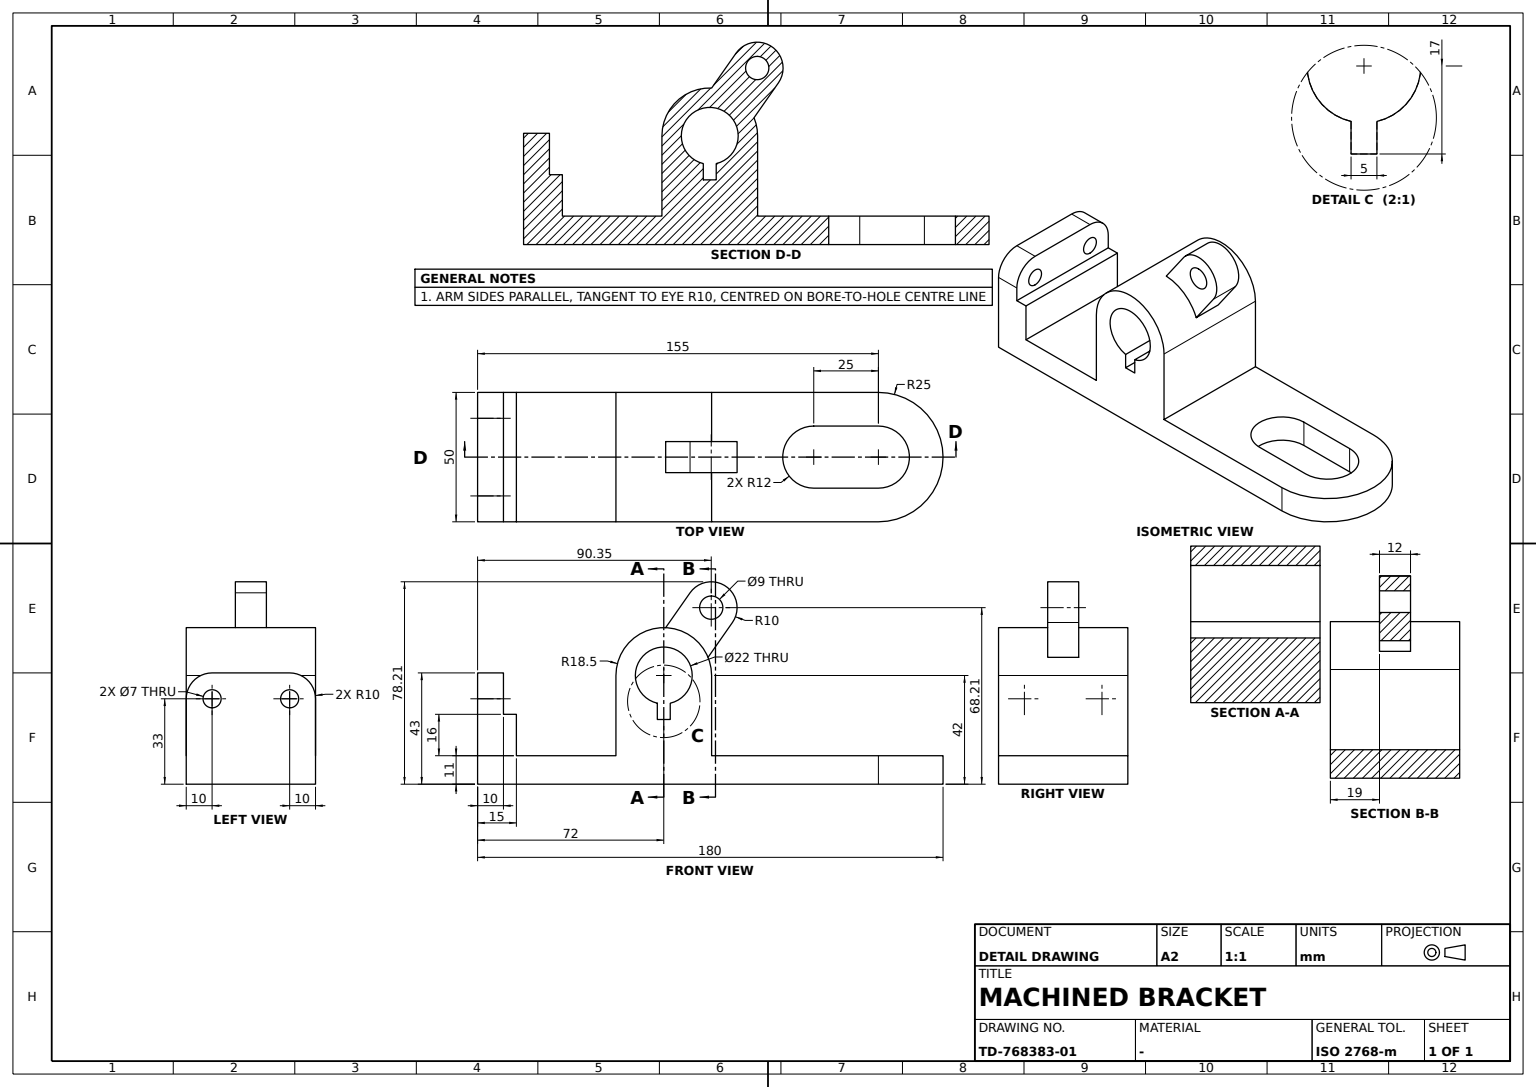
ISO-10303-21;
HEADER;
FILE_DESCRIPTION((''),'2;1');
FILE_NAME('','',(''),(''),'','','');
FILE_SCHEMA(('AUTOMOTIVE_DESIGN'));
ENDSEC;
DATA;
#1=APPLICATION_CONTEXT('');
#2=PRODUCT_CONTEXT('',#1,'mechanical');
#3=PRODUCT('','','',(#2));
#4=PRODUCT_DEFINITION_FORMATION('','',#3);
#5=PRODUCT_DEFINITION_CONTEXT('',#1,'design');
#6=PRODUCT_DEFINITION('','',#4,#5);
#7=PRODUCT_DEFINITION_SHAPE('','',#6);
#8=(LENGTH_UNIT()NAMED_UNIT(*)SI_UNIT(.MILLI.,.METRE.));
#9=(NAMED_UNIT(*)PLANE_ANGLE_UNIT()SI_UNIT($,.RADIAN.));
#10=(NAMED_UNIT(*)SI_UNIT($,.STERADIAN.)SOLID_ANGLE_UNIT());
#11=UNCERTAINTY_MEASURE_WITH_UNIT(LENGTH_MEASURE(0.005),#8,'distance_accuracy_value','');
#12=(GEOMETRIC_REPRESENTATION_CONTEXT(3)GLOBAL_UNCERTAINTY_ASSIGNED_CONTEXT((#11))GLOBAL_UNIT_ASSIGNED_CONTEXT((#8,#9,#10))REPRESENTATION_CONTEXT('',''));
#13=CARTESIAN_POINT('',(-77.5,15.,37.5));
#14=VERTEX_POINT('',#13);
#15=CARTESIAN_POINT('',(-77.5,25.,27.5));
#16=VERTEX_POINT('',#15);
#17=CARTESIAN_POINT('',(-77.5,15.,27.5));
#18=DIRECTION('',(1.,0.,0.));
#19=DIRECTION('',(0.,0.,-1.));
#20=AXIS2_PLACEMENT_3D('',#17,#18,#19);
#21=CIRCLE('',#20,10.);
#22=EDGE_CURVE('',#14,#16,#21,.F.);
#23=ORIENTED_EDGE('',*,*,#22,.F.);
#24=CARTESIAN_POINT('',(-67.5,15.,37.5));
#25=VERTEX_POINT('',#24);
#26=CARTESIAN_POINT('',(-70.,15.,37.5));
#27=DIRECTION('',(-1.,0.,0.));
#28=VECTOR('',#27,1000.);
#29=LINE('',#26,#28);
#30=EDGE_CURVE('',#14,#25,#29,.F.);
#31=ORIENTED_EDGE('',*,*,#30,.T.);
#32=CARTESIAN_POINT('',(-67.5,25.,27.5));
#33=VERTEX_POINT('',#32);
#34=CARTESIAN_POINT('',(-67.5,15.,27.5));
#35=AXIS2_PLACEMENT_3D('',#34,#18,#19);
#36=CIRCLE('',#35,10.);
#37=EDGE_CURVE('',#33,#25,#36,.T.);
#38=ORIENTED_EDGE('',*,*,#37,.F.);
#39=CARTESIAN_POINT('',(-70.,25.,27.5));
#40=LINE('',#39,#28);
#41=EDGE_CURVE('',#16,#33,#40,.F.);
#42=ORIENTED_EDGE('',*,*,#41,.F.);
#43=EDGE_LOOP('',(#23,#31,#38,#42));
#44=FACE_BOUND('',#43,.T.);
#45=CARTESIAN_POINT('',(-70.,15.,27.5));
#46=DIRECTION('',(0.,-1.,0.));
#47=AXIS2_PLACEMENT_3D('',#45,#27,#46);
#48=CYLINDRICAL_SURFACE('',#47,10.);
#49=ADVANCED_FACE('',(#44),#48,.T.);
#50=CARTESIAN_POINT('',(-67.5,-15.,24.));
#51=VERTEX_POINT('',#50);
#52=CARTESIAN_POINT('',(-67.5,-15.,27.5));
#53=AXIS2_PLACEMENT_3D('',#52,#18,#19);
#54=CIRCLE('',#53,3.5);
#55=EDGE_CURVE('',#51,#51,#54,.T.);
#56=ORIENTED_EDGE('',*,*,#55,.F.);
#57=EDGE_LOOP('',(#56));
#58=FACE_BOUND('',#57,.T.);
#59=CARTESIAN_POINT('',(-67.5,15.,24.));
#60=VERTEX_POINT('',#59);
#61=CIRCLE('',#35,3.5);
#62=EDGE_CURVE('',#60,#60,#61,.T.);
#63=ORIENTED_EDGE('',*,*,#62,.F.);
#64=EDGE_LOOP('',(#63));
#65=FACE_BOUND('',#64,.T.);
#66=CARTESIAN_POINT('',(-67.5,-15.,37.5));
#67=VERTEX_POINT('',#66);
#68=CARTESIAN_POINT('',(-67.5,-25.,27.5));
#69=VERTEX_POINT('',#68);
#70=CIRCLE('',#53,10.);
#71=EDGE_CURVE('',#67,#69,#70,.T.);
#72=ORIENTED_EDGE('',*,*,#71,.T.);
#73=CARTESIAN_POINT('',(-67.5,-25.,21.5));
#74=VERTEX_POINT('',#73);
#75=CARTESIAN_POINT('',(-67.5,-25.,0.));
#76=DIRECTION('',(0.,0.,1.));
#77=VECTOR('',#76,1000.);
#78=LINE('',#75,#77);
#79=EDGE_CURVE('',#74,#69,#78,.T.);
#80=ORIENTED_EDGE('',*,*,#79,.F.);
#81=CARTESIAN_POINT('',(-67.5,25.,21.5));
#82=VERTEX_POINT('',#81);
#83=VECTOR('',#46,1000.);
#84=LINE('',#81,#83);
#85=EDGE_CURVE('',#82,#74,#84,.T.);
#86=ORIENTED_EDGE('',*,*,#85,.F.);
#87=CARTESIAN_POINT('',(-67.5,25.,0.));
#88=VECTOR('',#19,1000.);
#89=LINE('',#87,#88);
#90=EDGE_CURVE('',#33,#82,#89,.T.);
#91=ORIENTED_EDGE('',*,*,#90,.F.);
#92=ORIENTED_EDGE('',*,*,#37,.T.);
#93=DIRECTION('',(0.,1.,0.));
#94=VECTOR('',#93,1000.);
#95=LINE('',#24,#94);
#96=EDGE_CURVE('',#67,#25,#95,.T.);
#97=ORIENTED_EDGE('',*,*,#96,.F.);
#98=EDGE_LOOP('',(#72,#80,#86,#91,#92,#97));
#99=FACE_BOUND('',#98,.T.);
#100=CARTESIAN_POINT('',(-67.5,0.,0.));
#101=AXIS2_PLACEMENT_3D('',#100,#18,#93);
#102=PLANE('',#101);
#103=ADVANCED_FACE('',(#58,#65,#99),#102,.T.);
#104=CARTESIAN_POINT('',(-24.,25.,5.5));
#105=VERTEX_POINT('',#104);
#106=CARTESIAN_POINT('',(-24.,25.,36.5));
#107=VERTEX_POINT('',#106);
#108=CARTESIAN_POINT('',(-24.,25.,-5.5));
#109=LINE('',#108,#77);
#110=EDGE_CURVE('',#105,#107,#109,.T.);
#111=ORIENTED_EDGE('',*,*,#110,.F.);
#112=CARTESIAN_POINT('',(-24.,-25.,5.5));
#113=VERTEX_POINT('',#112);
#114=CARTESIAN_POINT('',(-24.,0.,5.5));
#115=LINE('',#114,#83);
#116=EDGE_CURVE('',#105,#113,#115,.T.);
#117=ORIENTED_EDGE('',*,*,#116,.T.);
#118=CARTESIAN_POINT('',(-24.,-25.,36.5));
#119=VERTEX_POINT('',#118);
#120=CARTESIAN_POINT('',(-24.,-25.,0.));
#121=LINE('',#120,#77);
#122=EDGE_CURVE('',#113,#119,#121,.T.);
#123=ORIENTED_EDGE('',*,*,#122,.T.);
#124=CARTESIAN_POINT('',(-24.,0.,36.5));
#125=LINE('',#124,#83);
#126=EDGE_CURVE('',#119,#107,#125,.F.);
#127=ORIENTED_EDGE('',*,*,#126,.T.);
#128=EDGE_LOOP('',(#111,#117,#123,#127));
#129=FACE_BOUND('',#128,.T.);
#130=CARTESIAN_POINT('',(-24.,-25.,-5.5));
#131=AXIS2_PLACEMENT_3D('',#130,#27,#76);
#132=PLANE('',#131);
#133=ADVANCED_FACE('',(#129),#132,.T.);
#134=ORIENTED_EDGE('',*,*,#62,.T.);
#135=EDGE_LOOP('',(#134));
#136=FACE_BOUND('',#135,.T.);
#137=CARTESIAN_POINT('',(-77.5,15.,24.));
#138=VERTEX_POINT('',#137);
#139=CIRCLE('',#20,3.5);
#140=EDGE_CURVE('',#138,#138,#139,.T.);
#141=ORIENTED_EDGE('',*,*,#140,.F.);
#142=EDGE_LOOP('',(#141));
#143=FACE_BOUND('',#142,.T.);
#144=CARTESIAN_POINT('',(-73.16,15.,27.5));
#145=AXIS2_PLACEMENT_3D('',#144,#18,#93);
#146=CYLINDRICAL_SURFACE('',#145,3.5);
#147=ADVANCED_FACE('',(#136,#143),#146,.F.);
#148=CARTESIAN_POINT('',(-77.5,-15.,24.));
#149=VERTEX_POINT('',#148);
#150=CARTESIAN_POINT('',(-77.5,-15.,27.5));
#151=AXIS2_PLACEMENT_3D('',#150,#18,#19);
#152=CIRCLE('',#151,3.5);
#153=EDGE_CURVE('',#149,#149,#152,.T.);
#154=ORIENTED_EDGE('',*,*,#153,.F.);
#155=EDGE_LOOP('',(#154));
#156=FACE_BOUND('',#155,.T.);
#157=ORIENTED_EDGE('',*,*,#55,.T.);
#158=EDGE_LOOP('',(#157));
#159=FACE_BOUND('',#158,.T.);
#160=CARTESIAN_POINT('',(-73.16,-15.,27.5));
#161=AXIS2_PLACEMENT_3D('',#160,#18,#93);
#162=CYLINDRICAL_SURFACE('',#161,3.5);
#163=ADVANCED_FACE('',(#156,#159),#162,.F.);
#164=CARTESIAN_POINT('',(-8.,-25.,25.787857));
#165=VERTEX_POINT('',#164);
#166=CARTESIAN_POINT('',(-8.,-25.,19.5));
#167=VERTEX_POINT('',#166);
#168=LINE('',#164,#88);
#169=EDGE_CURVE('',#165,#167,#168,.T.);
#170=ORIENTED_EDGE('',*,*,#169,.T.);
#171=CARTESIAN_POINT('',(-8.,25.,19.5));
#172=VERTEX_POINT('',#171);
#173=CARTESIAN_POINT('',(-8.,6.,19.5));
#174=LINE('',#173,#83);
#175=EDGE_CURVE('',#172,#167,#174,.T.);
#176=ORIENTED_EDGE('',*,*,#175,.F.);
#177=CARTESIAN_POINT('',(-8.,25.,25.787857));
#178=VERTEX_POINT('',#177);
#179=CARTESIAN_POINT('',(-8.,25.,0.));
#180=LINE('',#179,#88);
#181=EDGE_CURVE('',#178,#172,#180,.T.);
#182=ORIENTED_EDGE('',*,*,#181,.F.);
#183=LINE('',#177,#94);
#184=EDGE_CURVE('',#178,#165,#183,.F.);
#185=ORIENTED_EDGE('',*,*,#184,.T.);
#186=EDGE_LOOP('',(#170,#176,#182,#185));
#187=FACE_BOUND('',#186,.T.);
#188=CARTESIAN_POINT('',(-8.,6.,25.787857));
#189=AXIS2_PLACEMENT_3D('',#188,#27,#19);
#190=PLANE('',#189);
#191=ADVANCED_FACE('',(#187),#190,.F.);
#192=CARTESIAN_POINT('',(-77.5,-15.,37.5));
#193=VERTEX_POINT('',#192);
#194=CARTESIAN_POINT('',(-70.,-15.,37.5));
#195=LINE('',#194,#28);
#196=EDGE_CURVE('',#193,#67,#195,.F.);
#197=ORIENTED_EDGE('',*,*,#196,.T.);
#198=ORIENTED_EDGE('',*,*,#96,.T.);
#199=ORIENTED_EDGE('',*,*,#30,.F.);
#200=CARTESIAN_POINT('',(-77.5,-25.,37.5));
#201=LINE('',#200,#83);
#202=EDGE_CURVE('',#14,#193,#201,.T.);
#203=ORIENTED_EDGE('',*,*,#202,.T.);
#204=EDGE_LOOP('',(#197,#198,#199,#203));
#205=FACE_BOUND('',#204,.T.);
#206=AXIS2_PLACEMENT_3D('',#13,#76,#46);
#207=PLANE('',#206);
#208=ADVANCED_FACE('',(#205),#207,.T.);
#209=ORIENTED_EDGE('',*,*,#140,.T.);
#210=EDGE_LOOP('',(#209));
#211=FACE_BOUND('',#210,.T.);
#212=CARTESIAN_POINT('',(-77.5,-25.,-5.5));
#213=VERTEX_POINT('',#212);
#214=CARTESIAN_POINT('',(-77.5,25.,-5.5));
#215=VERTEX_POINT('',#214);
#216=CARTESIAN_POINT('',(-77.5,0.,-5.5));
#217=LINE('',#216,#94);
#218=EDGE_CURVE('',#213,#215,#217,.T.);
#219=ORIENTED_EDGE('',*,*,#218,.F.);
#220=CARTESIAN_POINT('',(-77.5,-25.,27.5));
#221=VERTEX_POINT('',#220);
#222=CARTESIAN_POINT('',(-77.5,-25.,0.));
#223=LINE('',#222,#88);
#224=EDGE_CURVE('',#221,#213,#223,.T.);
#225=ORIENTED_EDGE('',*,*,#224,.F.);
#226=CIRCLE('',#151,10.);
#227=EDGE_CURVE('',#221,#193,#226,.F.);
#228=ORIENTED_EDGE('',*,*,#227,.T.);
#229=ORIENTED_EDGE('',*,*,#202,.F.);
#230=ORIENTED_EDGE('',*,*,#22,.T.);
#231=CARTESIAN_POINT('',(-77.5,25.,0.));
#232=LINE('',#231,#77);
#233=EDGE_CURVE('',#215,#16,#232,.T.);
#234=ORIENTED_EDGE('',*,*,#233,.F.);
#235=EDGE_LOOP('',(#219,#225,#228,#229,#230,#234));
#236=FACE_BOUND('',#235,.T.);
#237=ORIENTED_EDGE('',*,*,#153,.T.);
#238=EDGE_LOOP('',(#237));
#239=FACE_BOUND('',#238,.T.);
#240=AXIS2_PLACEMENT_3D('',#222,#18,#93);
#241=PLANE('',#240);
#242=ADVANCED_FACE('',(#211,#236,#239),#241,.F.);
#243=CARTESIAN_POINT('',(-3.,-25.,19.5));
#244=VERTEX_POINT('',#243);
#245=LINE('',#243,#28);
#246=EDGE_CURVE('',#244,#167,#245,.T.);
#247=ORIENTED_EDGE('',*,*,#246,.T.);
#248=ORIENTED_EDGE('',*,*,#169,.F.);
#249=CARTESIAN_POINT('',(-3.,-25.,25.787857));
#250=VERTEX_POINT('',#249);
#251=CARTESIAN_POINT('',(-5.5,-25.,36.5));
#252=AXIS2_PLACEMENT_3D('',#251,#93,#76);
#253=CIRCLE('',#252,11.);
#254=EDGE_CURVE('',#165,#250,#253,.T.);
#255=ORIENTED_EDGE('',*,*,#254,.T.);
#256=LINE('',#249,#88);
#257=EDGE_CURVE('',#250,#244,#256,.T.);
#258=ORIENTED_EDGE('',*,*,#257,.T.);
#259=EDGE_LOOP('',(#247,#248,#255,#258));
#260=FACE_BOUND('',#259,.T.);
#261=ORIENTED_EDGE('',*,*,#79,.T.);
#262=CARTESIAN_POINT('',(-70.,-25.,27.5));
#263=LINE('',#262,#28);
#264=EDGE_CURVE('',#221,#69,#263,.F.);
#265=ORIENTED_EDGE('',*,*,#264,.F.);
#266=ORIENTED_EDGE('',*,*,#224,.T.);
#267=CARTESIAN_POINT('',(77.5,-25.,-5.5));
#268=VERTEX_POINT('',#267);
#269=CARTESIAN_POINT('',(0.,-25.,-5.5));
#270=LINE('',#269,#28);
#271=EDGE_CURVE('',#268,#213,#270,.T.);
#272=ORIENTED_EDGE('',*,*,#271,.F.);
#273=CARTESIAN_POINT('',(77.5,-25.,5.5));
#274=VERTEX_POINT('',#273);
#275=CARTESIAN_POINT('',(77.5,-25.,0.));
#276=LINE('',#275,#77);
#277=EDGE_CURVE('',#268,#274,#276,.T.);
#278=ORIENTED_EDGE('',*,*,#277,.T.);
#279=CARTESIAN_POINT('',(13.,-25.,5.5));
#280=VERTEX_POINT('',#279);
#281=CARTESIAN_POINT('',(0.,-25.,5.5));
#282=LINE('',#281,#28);
#283=EDGE_CURVE('',#274,#280,#282,.T.);
#284=ORIENTED_EDGE('',*,*,#283,.T.);
#285=CARTESIAN_POINT('',(13.,-25.,36.5));
#286=VERTEX_POINT('',#285);
#287=CARTESIAN_POINT('',(13.,-25.,0.));
#288=LINE('',#287,#88);
#289=EDGE_CURVE('',#286,#280,#288,.T.);
#290=ORIENTED_EDGE('',*,*,#289,.F.);
#291=CIRCLE('',#252,18.5);
#292=EDGE_CURVE('',#286,#119,#291,.F.);
#293=ORIENTED_EDGE('',*,*,#292,.T.);
#294=ORIENTED_EDGE('',*,*,#122,.F.);
#295=CARTESIAN_POINT('',(-62.5,-25.,5.5));
#296=VERTEX_POINT('',#295);
#297=EDGE_CURVE('',#113,#296,#282,.T.);
#298=ORIENTED_EDGE('',*,*,#297,.T.);
#299=CARTESIAN_POINT('',(-62.5,-25.,21.5));
#300=VERTEX_POINT('',#299);
#301=CARTESIAN_POINT('',(-62.5,-25.,0.));
#302=LINE('',#301,#88);
#303=EDGE_CURVE('',#300,#296,#302,.T.);
#304=ORIENTED_EDGE('',*,*,#303,.F.);
#305=CARTESIAN_POINT('',(77.5,-25.,21.5));
#306=LINE('',#305,#28);
#307=EDGE_CURVE('',#300,#74,#306,.T.);
#308=ORIENTED_EDGE('',*,*,#307,.T.);
#309=EDGE_LOOP('',(#261,#265,#266,#272,#278,#284,#290,#293,#294,#298,#304,#308));
#310=FACE_BOUND('',#309,.T.);
#311=AXIS2_PLACEMENT_3D('',#275,#93,#27);
#312=PLANE('',#311);
#313=ADVANCED_FACE('',(#260,#310),#312,.F.);
#314=ORIENTED_EDGE('',*,*,#303,.T.);
#315=CARTESIAN_POINT('',(-62.5,25.,5.5));
#316=VERTEX_POINT('',#315);
#317=CARTESIAN_POINT('',(-62.5,0.,5.5));
#318=LINE('',#317,#83);
#319=EDGE_CURVE('',#316,#296,#318,.T.);
#320=ORIENTED_EDGE('',*,*,#319,.F.);
#321=CARTESIAN_POINT('',(-62.5,25.,21.5));
#322=VERTEX_POINT('',#321);
#323=CARTESIAN_POINT('',(-62.5,25.,0.));
#324=LINE('',#323,#77);
#325=EDGE_CURVE('',#316,#322,#324,.T.);
#326=ORIENTED_EDGE('',*,*,#325,.T.);
#327=CARTESIAN_POINT('',(-62.5,0.,21.5));
#328=LINE('',#327,#83);
#329=EDGE_CURVE('',#322,#300,#328,.T.);
#330=ORIENTED_EDGE('',*,*,#329,.T.);
#331=EDGE_LOOP('',(#314,#320,#326,#330));
#332=FACE_BOUND('',#331,.T.);
#333=CARTESIAN_POINT('',(-62.5,0.,0.));
#334=AXIS2_PLACEMENT_3D('',#333,#27,#46);
#335=PLANE('',#334);
#336=ADVANCED_FACE('',(#332),#335,.F.);
#337=ORIENTED_EDGE('',*,*,#116,.F.);
#338=CARTESIAN_POINT('',(0.,25.,5.5));
#339=VECTOR('',#18,1000.);
#340=LINE('',#338,#339);
#341=EDGE_CURVE('',#316,#105,#340,.T.);
#342=ORIENTED_EDGE('',*,*,#341,.F.);
#343=ORIENTED_EDGE('',*,*,#319,.T.);
#344=ORIENTED_EDGE('',*,*,#297,.F.);
#345=EDGE_LOOP('',(#337,#342,#343,#344));
#346=FACE_BOUND('',#345,.T.);
#347=CARTESIAN_POINT('',(0.,0.,5.5));
#348=AXIS2_PLACEMENT_3D('',#347,#76,#18);
#349=PLANE('',#348);
#350=ADVANCED_FACE('',(#346),#349,.T.);
#351=CARTESIAN_POINT('',(-3.,25.,25.787857));
#352=VERTEX_POINT('',#351);
#353=CARTESIAN_POINT('',(-3.,25.,19.5));
#354=VERTEX_POINT('',#353);
#355=CARTESIAN_POINT('',(-3.,25.,0.));
#356=LINE('',#355,#88);
#357=EDGE_CURVE('',#352,#354,#356,.T.);
#358=ORIENTED_EDGE('',*,*,#357,.T.);
#359=CARTESIAN_POINT('',(-3.,6.,19.5));
#360=LINE('',#359,#83);
#361=EDGE_CURVE('',#354,#244,#360,.T.);
#362=ORIENTED_EDGE('',*,*,#361,.T.);
#363=ORIENTED_EDGE('',*,*,#257,.F.);
#364=LINE('',#351,#94);
#365=EDGE_CURVE('',#352,#250,#364,.F.);
#366=ORIENTED_EDGE('',*,*,#365,.F.);
#367=EDGE_LOOP('',(#358,#362,#363,#366));
#368=FACE_BOUND('',#367,.T.);
#369=CARTESIAN_POINT('',(-3.,6.,25.787857));
#370=AXIS2_PLACEMENT_3D('',#369,#27,#19);
#371=PLANE('',#370);
#372=ADVANCED_FACE('',(#368),#371,.T.);
#373=CARTESIAN_POINT('',(77.5,-12.,-5.5));
#374=VERTEX_POINT('',#373);
#375=CARTESIAN_POINT('',(52.5,-12.,-5.5));
#376=VERTEX_POINT('',#375);
#377=LINE('',#373,#28);
#378=EDGE_CURVE('',#374,#376,#377,.T.);
#379=ORIENTED_EDGE('',*,*,#378,.T.);
#380=CARTESIAN_POINT('',(52.5,-12.,5.5));
#381=VERTEX_POINT('',#380);
#382=CARTESIAN_POINT('',(52.5,-12.,-0.66));
#383=LINE('',#382,#77);
#384=EDGE_CURVE('',#381,#376,#383,.F.);
#385=ORIENTED_EDGE('',*,*,#384,.F.);
#386=CARTESIAN_POINT('',(77.5,-12.,5.5));
#387=VERTEX_POINT('',#386);
#388=LINE('',#386,#28);
#389=EDGE_CURVE('',#387,#381,#388,.T.);
#390=ORIENTED_EDGE('',*,*,#389,.F.);
#391=CARTESIAN_POINT('',(77.5,-12.,-0.66));
#392=LINE('',#391,#77);
#393=EDGE_CURVE('',#387,#374,#392,.F.);
#394=ORIENTED_EDGE('',*,*,#393,.T.);
#395=EDGE_LOOP('',(#379,#385,#390,#394));
#396=FACE_BOUND('',#395,.T.);
#397=AXIS2_PLACEMENT_3D('',#386,#46,#27);
#398=PLANE('',#397);
#399=ADVANCED_FACE('',(#396),#398,.F.);
#400=ORIENTED_EDGE('',*,*,#307,.F.);
#401=ORIENTED_EDGE('',*,*,#329,.F.);
#402=LINE('',#321,#28);
#403=EDGE_CURVE('',#322,#82,#402,.T.);
#404=ORIENTED_EDGE('',*,*,#403,.T.);
#405=ORIENTED_EDGE('',*,*,#85,.T.);
#406=EDGE_LOOP('',(#400,#401,#404,#405));
#407=FACE_BOUND('',#406,.T.);
#408=AXIS2_PLACEMENT_3D('',#321,#19,#46);
#409=PLANE('',#408);
#410=ADVANCED_FACE('',(#407),#409,.F.);
#411=CARTESIAN_POINT('',(52.5,12.,5.5));
#412=VERTEX_POINT('',#411);
#413=CARTESIAN_POINT('',(52.5,12.,-5.5));
#414=VERTEX_POINT('',#413);
#415=CARTESIAN_POINT('',(52.5,12.,-0.66));
#416=LINE('',#415,#77);
#417=EDGE_CURVE('',#412,#414,#416,.F.);
#418=ORIENTED_EDGE('',*,*,#417,.T.);
#419=CARTESIAN_POINT('',(77.5,12.,-5.5));
#420=VERTEX_POINT('',#419);
#421=LINE('',#413,#339);
#422=EDGE_CURVE('',#414,#420,#421,.T.);
#423=ORIENTED_EDGE('',*,*,#422,.T.);
#424=CARTESIAN_POINT('',(77.5,12.,5.5));
#425=VERTEX_POINT('',#424);
#426=CARTESIAN_POINT('',(77.5,12.,-0.66));
#427=LINE('',#426,#77);
#428=EDGE_CURVE('',#425,#420,#427,.F.);
#429=ORIENTED_EDGE('',*,*,#428,.F.);
#430=LINE('',#411,#339);
#431=EDGE_CURVE('',#412,#425,#430,.T.);
#432=ORIENTED_EDGE('',*,*,#431,.F.);
#433=EDGE_LOOP('',(#418,#423,#429,#432));
#434=FACE_BOUND('',#433,.T.);
#435=AXIS2_PLACEMENT_3D('',#411,#93,#18);
#436=PLANE('',#435);
#437=ADVANCED_FACE('',(#434),#436,.F.);
#438=CARTESIAN_POINT('',(11.618883,-6.,43.513831));
#439=VERTEX_POINT('',#438);
#440=CARTESIAN_POINT('',(21.045966,-6.,56.977101));
#441=VERTEX_POINT('',#440);
#442=CARTESIAN_POINT('',(-12.648425,-6.,8.856523));
#443=DIRECTION('',(0.573576436,0.,0.819152044));
#444=VECTOR('',#443,1000.);
#445=LINE('',#442,#444);
#446=EDGE_CURVE('',#439,#441,#445,.T.);
#447=ORIENTED_EDGE('',*,*,#446,.T.);
#448=CARTESIAN_POINT('',(4.662926,-6.,68.44863));
#449=VERTEX_POINT('',#448);
#450=CARTESIAN_POINT('',(12.854446,-6.,62.712865));
#451=AXIS2_PLACEMENT_3D('',#450,#93,#76);
#452=CIRCLE('',#451,10.);
#453=EDGE_CURVE('',#449,#441,#452,.T.);
#454=ORIENTED_EDGE('',*,*,#453,.F.);
#455=CARTESIAN_POINT('',(-4.764157,-6.,54.98536));
#456=VERTEX_POINT('',#455);
#457=CARTESIAN_POINT('',(-29.031466,-6.,20.328051));
#458=LINE('',#457,#444);
#459=EDGE_CURVE('',#456,#449,#458,.T.);
#460=ORIENTED_EDGE('',*,*,#459,.F.);
#461=CARTESIAN_POINT('',(-5.5,-6.,36.5));
#462=AXIS2_PLACEMENT_3D('',#461,#93,#76);
#463=CIRCLE('',#462,18.5);
#464=EDGE_CURVE('',#456,#439,#463,.T.);
#465=ORIENTED_EDGE('',*,*,#464,.T.);
#466=EDGE_LOOP('',(#447,#454,#460,#465));
#467=FACE_BOUND('',#466,.T.);
#468=CARTESIAN_POINT('',(12.854446,-6.,67.212865));
#469=VERTEX_POINT('',#468);
#470=CIRCLE('',#451,4.5);
#471=EDGE_CURVE('',#469,#469,#470,.T.);
#472=ORIENTED_EDGE('',*,*,#471,.T.);
#473=EDGE_LOOP('',(#472));
#474=FACE_BOUND('',#473,.T.);
#475=CARTESIAN_POINT('',(0.,-6.,0.));
#476=AXIS2_PLACEMENT_3D('',#475,#93,#27);
#477=PLANE('',#476);
#478=ADVANCED_FACE('',(#467,#474),#477,.F.);
#479=CARTESIAN_POINT('',(-4.764157,6.,54.98536));
#480=VERTEX_POINT('',#479);
#481=LINE('',#455,#83);
#482=EDGE_CURVE('',#456,#480,#481,.F.);
#483=ORIENTED_EDGE('',*,*,#482,.T.);
#484=CARTESIAN_POINT('',(11.618883,6.,43.513831));
#485=VERTEX_POINT('',#484);
#486=CARTESIAN_POINT('',(-5.5,6.,36.5));
#487=AXIS2_PLACEMENT_3D('',#486,#93,#76);
#488=CIRCLE('',#487,18.5);
#489=EDGE_CURVE('',#480,#485,#488,.T.);
#490=ORIENTED_EDGE('',*,*,#489,.T.);
#491=LINE('',#438,#83);
#492=EDGE_CURVE('',#439,#485,#491,.F.);
#493=ORIENTED_EDGE('',*,*,#492,.F.);
#494=ORIENTED_EDGE('',*,*,#464,.F.);
#495=EDGE_LOOP('',(#483,#490,#493,#494));
#496=FACE_BOUND('',#495,.T.);
#497=ORIENTED_EDGE('',*,*,#126,.F.);
#498=ORIENTED_EDGE('',*,*,#292,.F.);
#499=CARTESIAN_POINT('',(13.,25.,36.5));
#500=VERTEX_POINT('',#499);
#501=CARTESIAN_POINT('',(13.,0.,36.5));
#502=LINE('',#501,#83);
#503=EDGE_CURVE('',#286,#500,#502,.F.);
#504=ORIENTED_EDGE('',*,*,#503,.T.);
#505=CARTESIAN_POINT('',(-5.5,25.,36.5));
#506=AXIS2_PLACEMENT_3D('',#505,#46,#19);
#507=CIRCLE('',#506,18.5);
#508=EDGE_CURVE('',#500,#107,#507,.T.);
#509=ORIENTED_EDGE('',*,*,#508,.T.);
#510=EDGE_LOOP('',(#497,#498,#504,#509));
#511=FACE_BOUND('',#510,.T.);
#512=CARTESIAN_POINT('',(-5.5,0.,36.5));
#513=AXIS2_PLACEMENT_3D('',#512,#46,#18);
#514=CYLINDRICAL_SURFACE('',#513,18.5);
#515=ADVANCED_FACE('',(#496,#511),#514,.T.);
#516=CARTESIAN_POINT('',(77.5,0.,5.5));
#517=AXIS2_PLACEMENT_3D('',#516,#76,#18);
#518=CIRCLE('',#517,12.);
#519=EDGE_CURVE('',#387,#425,#518,.T.);
#520=ORIENTED_EDGE('',*,*,#519,.F.);
#521=ORIENTED_EDGE('',*,*,#389,.T.);
#522=CARTESIAN_POINT('',(52.5,0.,5.5));
#523=AXIS2_PLACEMENT_3D('',#522,#76,#18);
#524=CIRCLE('',#523,12.);
#525=EDGE_CURVE('',#412,#381,#524,.T.);
#526=ORIENTED_EDGE('',*,*,#525,.F.);
#527=ORIENTED_EDGE('',*,*,#431,.T.);
#528=EDGE_LOOP('',(#520,#521,#526,#527));
#529=FACE_BOUND('',#528,.T.);
#530=CARTESIAN_POINT('',(13.,25.,5.5));
#531=VERTEX_POINT('',#530);
#532=CARTESIAN_POINT('',(77.5,25.,5.5));
#533=VERTEX_POINT('',#532);
#534=EDGE_CURVE('',#531,#533,#340,.T.);
#535=ORIENTED_EDGE('',*,*,#534,.F.);
#536=LINE('',#279,#83);
#537=EDGE_CURVE('',#531,#280,#536,.T.);
#538=ORIENTED_EDGE('',*,*,#537,.T.);
#539=ORIENTED_EDGE('',*,*,#283,.F.);
#540=CIRCLE('',#517,25.);
#541=EDGE_CURVE('',#274,#533,#540,.T.);
#542=ORIENTED_EDGE('',*,*,#541,.T.);
#543=EDGE_LOOP('',(#535,#538,#539,#542));
#544=FACE_BOUND('',#543,.T.);
#545=ADVANCED_FACE('',(#529,#544),#349,.T.);
#546=ORIENTED_EDGE('',*,*,#422,.F.);
#547=CARTESIAN_POINT('',(52.5,0.,-5.5));
#548=AXIS2_PLACEMENT_3D('',#547,#76,#18);
#549=CIRCLE('',#548,12.);
#550=EDGE_CURVE('',#414,#376,#549,.T.);
#551=ORIENTED_EDGE('',*,*,#550,.T.);
#552=ORIENTED_EDGE('',*,*,#378,.F.);
#553=CARTESIAN_POINT('',(77.5,0.,-5.5));
#554=AXIS2_PLACEMENT_3D('',#553,#76,#18);
#555=CIRCLE('',#554,12.);
#556=EDGE_CURVE('',#374,#420,#555,.T.);
#557=ORIENTED_EDGE('',*,*,#556,.T.);
#558=EDGE_LOOP('',(#546,#551,#552,#557));
#559=FACE_BOUND('',#558,.T.);
#560=ORIENTED_EDGE('',*,*,#271,.T.);
#561=ORIENTED_EDGE('',*,*,#218,.T.);
#562=CARTESIAN_POINT('',(77.5,25.,-5.5));
#563=VERTEX_POINT('',#562);
#564=CARTESIAN_POINT('',(0.,25.,-5.5));
#565=LINE('',#564,#339);
#566=EDGE_CURVE('',#215,#563,#565,.T.);
#567=ORIENTED_EDGE('',*,*,#566,.T.);
#568=CIRCLE('',#554,25.);
#569=EDGE_CURVE('',#268,#563,#568,.T.);
#570=ORIENTED_EDGE('',*,*,#569,.F.);
#571=EDGE_LOOP('',(#560,#561,#567,#570));
#572=FACE_BOUND('',#571,.T.);
#573=CARTESIAN_POINT('',(0.,0.,-5.5));
#574=AXIS2_PLACEMENT_3D('',#573,#76,#18);
#575=PLANE('',#574);
#576=ADVANCED_FACE('',(#559,#572),#575,.F.);
#577=ORIENTED_EDGE('',*,*,#289,.T.);
#578=ORIENTED_EDGE('',*,*,#537,.F.);
#579=LINE('',#499,#88);
#580=EDGE_CURVE('',#500,#531,#579,.T.);
#581=ORIENTED_EDGE('',*,*,#580,.F.);
#582=ORIENTED_EDGE('',*,*,#503,.F.);
#583=EDGE_LOOP('',(#577,#578,#581,#582));
#584=FACE_BOUND('',#583,.T.);
#585=AXIS2_PLACEMENT_3D('',#285,#18,#19);
#586=PLANE('',#585);
#587=ADVANCED_FACE('',(#584),#586,.T.);
#588=CARTESIAN_POINT('',(21.045966,6.,56.977101));
#589=VERTEX_POINT('',#588);
#590=CARTESIAN_POINT('',(-12.648425,6.,8.856523));
#591=LINE('',#590,#444);
#592=EDGE_CURVE('',#485,#589,#591,.T.);
#593=ORIENTED_EDGE('',*,*,#592,.T.);
#594=CARTESIAN_POINT('',(21.045966,0.,56.977101));
#595=LINE('',#594,#94);
#596=EDGE_CURVE('',#441,#589,#595,.T.);
#597=ORIENTED_EDGE('',*,*,#596,.F.);
#598=ORIENTED_EDGE('',*,*,#446,.F.);
#599=ORIENTED_EDGE('',*,*,#492,.T.);
#600=EDGE_LOOP('',(#593,#597,#598,#599));
#601=FACE_BOUND('',#600,.T.);
#602=CARTESIAN_POINT('',(11.618883,0.,43.513831));
#603=DIRECTION('',(-0.819152044,0.,0.573576436));
#604=AXIS2_PLACEMENT_3D('',#602,#603,#443);
#605=PLANE('',#604);
#606=ADVANCED_FACE('',(#601),#605,.F.);
#607=CARTESIAN_POINT('',(4.662926,6.,68.44863));
#608=VERTEX_POINT('',#607);
#609=CARTESIAN_POINT('',(-29.031466,6.,20.328051));
#610=LINE('',#609,#444);
#611=EDGE_CURVE('',#480,#608,#610,.T.);
#612=ORIENTED_EDGE('',*,*,#611,.F.);
#613=ORIENTED_EDGE('',*,*,#482,.F.);
#614=ORIENTED_EDGE('',*,*,#459,.T.);
#615=CARTESIAN_POINT('',(4.662926,0.,68.44863));
#616=LINE('',#615,#94);
#617=EDGE_CURVE('',#449,#608,#616,.T.);
#618=ORIENTED_EDGE('',*,*,#617,.T.);
#619=EDGE_LOOP('',(#612,#613,#614,#618));
#620=FACE_BOUND('',#619,.T.);
#621=CARTESIAN_POINT('',(-4.764157,0.,54.98536));
#622=AXIS2_PLACEMENT_3D('',#621,#603,#443);
#623=PLANE('',#622);
#624=ADVANCED_FACE('',(#620),#623,.T.);
#625=ORIENTED_EDGE('',*,*,#254,.F.);
#626=ORIENTED_EDGE('',*,*,#184,.F.);
#627=CIRCLE('',#506,11.);
#628=EDGE_CURVE('',#352,#178,#627,.T.);
#629=ORIENTED_EDGE('',*,*,#628,.F.);
#630=ORIENTED_EDGE('',*,*,#365,.T.);
#631=EDGE_LOOP('',(#625,#626,#629,#630));
#632=FACE_BOUND('',#631,.T.);
#633=CARTESIAN_POINT('',(-5.5,-10.16,36.5));
#634=AXIS2_PLACEMENT_3D('',#633,#93,#27);
#635=CYLINDRICAL_SURFACE('',#634,11.);
#636=ADVANCED_FACE('',(#632),#635,.F.);
#637=ORIENTED_EDGE('',*,*,#471,.F.);
#638=EDGE_LOOP('',(#637));
#639=FACE_BOUND('',#638,.T.);
#640=CARTESIAN_POINT('',(12.854446,6.,67.212865));
#641=VERTEX_POINT('',#640);
#642=CARTESIAN_POINT('',(12.854446,6.,62.712865));
#643=AXIS2_PLACEMENT_3D('',#642,#93,#76);
#644=CIRCLE('',#643,4.5);
#645=EDGE_CURVE('',#641,#641,#644,.T.);
#646=ORIENTED_EDGE('',*,*,#645,.T.);
#647=EDGE_LOOP('',(#646));
#648=FACE_BOUND('',#647,.T.);
#649=CARTESIAN_POINT('',(12.854446,-10.16,62.712865));
#650=AXIS2_PLACEMENT_3D('',#649,#93,#27);
#651=CYLINDRICAL_SURFACE('',#650,4.5);
#652=ADVANCED_FACE('',(#639,#648),#651,.F.);
#653=ORIENTED_EDGE('',*,*,#181,.T.);
#654=CARTESIAN_POINT('',(-77.5,25.,19.5));
#655=LINE('',#654,#28);
#656=EDGE_CURVE('',#354,#172,#655,.T.);
#657=ORIENTED_EDGE('',*,*,#656,.F.);
#658=ORIENTED_EDGE('',*,*,#357,.F.);
#659=ORIENTED_EDGE('',*,*,#628,.T.);
#660=EDGE_LOOP('',(#653,#657,#658,#659));
#661=FACE_BOUND('',#660,.T.);
#662=ORIENTED_EDGE('',*,*,#325,.F.);
#663=ORIENTED_EDGE('',*,*,#341,.T.);
#664=ORIENTED_EDGE('',*,*,#110,.T.);
#665=ORIENTED_EDGE('',*,*,#508,.F.);
#666=ORIENTED_EDGE('',*,*,#580,.T.);
#667=ORIENTED_EDGE('',*,*,#534,.T.);
#668=CARTESIAN_POINT('',(77.5,25.,0.));
#669=LINE('',#668,#77);
#670=EDGE_CURVE('',#563,#533,#669,.T.);
#671=ORIENTED_EDGE('',*,*,#670,.F.);
#672=ORIENTED_EDGE('',*,*,#566,.F.);
#673=ORIENTED_EDGE('',*,*,#233,.T.);
#674=ORIENTED_EDGE('',*,*,#41,.T.);
#675=ORIENTED_EDGE('',*,*,#90,.T.);
#676=ORIENTED_EDGE('',*,*,#403,.F.);
#677=EDGE_LOOP('',(#662,#663,#664,#665,#666,#667,#671,#672,#673,#674,#675,#676));
#678=FACE_BOUND('',#677,.T.);
#679=AXIS2_PLACEMENT_3D('',#231,#46,#18);
#680=PLANE('',#679);
#681=ADVANCED_FACE('',(#661,#678),#680,.F.);
#682=ORIENTED_EDGE('',*,*,#617,.F.);
#683=ORIENTED_EDGE('',*,*,#453,.T.);
#684=ORIENTED_EDGE('',*,*,#596,.T.);
#685=CIRCLE('',#643,10.);
#686=EDGE_CURVE('',#608,#589,#685,.T.);
#687=ORIENTED_EDGE('',*,*,#686,.F.);
#688=EDGE_LOOP('',(#682,#683,#684,#687));
#689=FACE_BOUND('',#688,.T.);
#690=CARTESIAN_POINT('',(12.854446,0.,62.712865));
#691=AXIS2_PLACEMENT_3D('',#690,#93,#27);
#692=CYLINDRICAL_SURFACE('',#691,10.);
#693=ADVANCED_FACE('',(#689),#692,.T.);
#694=ORIENTED_EDGE('',*,*,#246,.F.);
#695=ORIENTED_EDGE('',*,*,#361,.F.);
#696=ORIENTED_EDGE('',*,*,#656,.T.);
#697=ORIENTED_EDGE('',*,*,#175,.T.);
#698=EDGE_LOOP('',(#694,#695,#696,#697));
#699=FACE_BOUND('',#698,.T.);
#700=AXIS2_PLACEMENT_3D('',#359,#76,#27);
#701=PLANE('',#700);
#702=ADVANCED_FACE('',(#699),#701,.T.);
#703=ORIENTED_EDGE('',*,*,#417,.F.);
#704=ORIENTED_EDGE('',*,*,#525,.T.);
#705=ORIENTED_EDGE('',*,*,#384,.T.);
#706=ORIENTED_EDGE('',*,*,#550,.F.);
#707=EDGE_LOOP('',(#703,#704,#705,#706));
#708=FACE_BOUND('',#707,.T.);
#709=CARTESIAN_POINT('',(52.5,0.,-0.66));
#710=AXIS2_PLACEMENT_3D('',#709,#76,#18);
#711=CYLINDRICAL_SURFACE('',#710,12.);
#712=ADVANCED_FACE('',(#708),#711,.F.);
#713=ORIENTED_EDGE('',*,*,#393,.F.);
#714=ORIENTED_EDGE('',*,*,#519,.T.);
#715=ORIENTED_EDGE('',*,*,#428,.T.);
#716=ORIENTED_EDGE('',*,*,#556,.F.);
#717=EDGE_LOOP('',(#713,#714,#715,#716));
#718=FACE_BOUND('',#717,.T.);
#719=CARTESIAN_POINT('',(77.5,0.,-0.66));
#720=AXIS2_PLACEMENT_3D('',#719,#76,#18);
#721=CYLINDRICAL_SURFACE('',#720,12.);
#722=ADVANCED_FACE('',(#718),#721,.F.);
#723=ORIENTED_EDGE('',*,*,#264,.T.);
#724=ORIENTED_EDGE('',*,*,#71,.F.);
#725=ORIENTED_EDGE('',*,*,#196,.F.);
#726=ORIENTED_EDGE('',*,*,#227,.F.);
#727=EDGE_LOOP('',(#723,#724,#725,#726));
#728=FACE_BOUND('',#727,.T.);
#729=CARTESIAN_POINT('',(-70.,-15.,27.5));
#730=AXIS2_PLACEMENT_3D('',#729,#27,#46);
#731=CYLINDRICAL_SURFACE('',#730,10.);
#732=ADVANCED_FACE('',(#728),#731,.T.);
#733=ORIENTED_EDGE('',*,*,#277,.F.);
#734=ORIENTED_EDGE('',*,*,#569,.T.);
#735=ORIENTED_EDGE('',*,*,#670,.T.);
#736=ORIENTED_EDGE('',*,*,#541,.F.);
#737=EDGE_LOOP('',(#733,#734,#735,#736));
#738=FACE_BOUND('',#737,.T.);
#739=CARTESIAN_POINT('',(77.5,0.,0.));
#740=AXIS2_PLACEMENT_3D('',#739,#76,#18);
#741=CYLINDRICAL_SURFACE('',#740,25.);
#742=ADVANCED_FACE('',(#738),#741,.T.);
#743=ORIENTED_EDGE('',*,*,#645,.F.);
#744=EDGE_LOOP('',(#743));
#745=FACE_BOUND('',#744,.T.);
#746=ORIENTED_EDGE('',*,*,#611,.T.);
#747=ORIENTED_EDGE('',*,*,#686,.T.);
#748=ORIENTED_EDGE('',*,*,#592,.F.);
#749=ORIENTED_EDGE('',*,*,#489,.F.);
#750=EDGE_LOOP('',(#746,#747,#748,#749));
#751=FACE_BOUND('',#750,.T.);
#752=CARTESIAN_POINT('',(0.,6.,0.));
#753=AXIS2_PLACEMENT_3D('',#752,#93,#27);
#754=PLANE('',#753);
#755=ADVANCED_FACE('',(#745,#751),#754,.T.);
#756=CLOSED_SHELL('',(#49,#103,#133,#147,#163,#191,#208,#242,#313,#336,#350,#372,#399,#410,#437,#478,#515,#545,#576,#587,#606,#624,#636,#652,#681,#693,#702,#712,#722,#732,#742,#755));
#757=MANIFOLD_SOLID_BREP('',#756);
#758=ADVANCED_BREP_SHAPE_REPRESENTATION('',(#757),#12);
#759=SHAPE_DEFINITION_REPRESENTATION(#7,#758);
ENDSEC;
END-ISO-10303-21;
